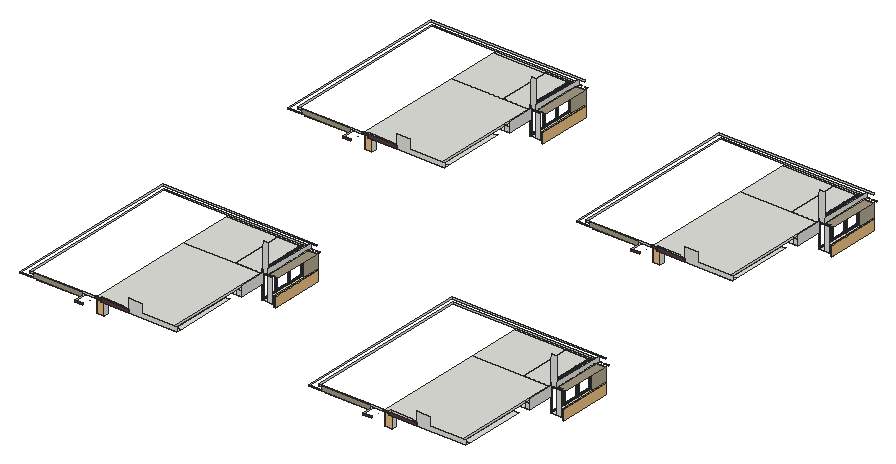
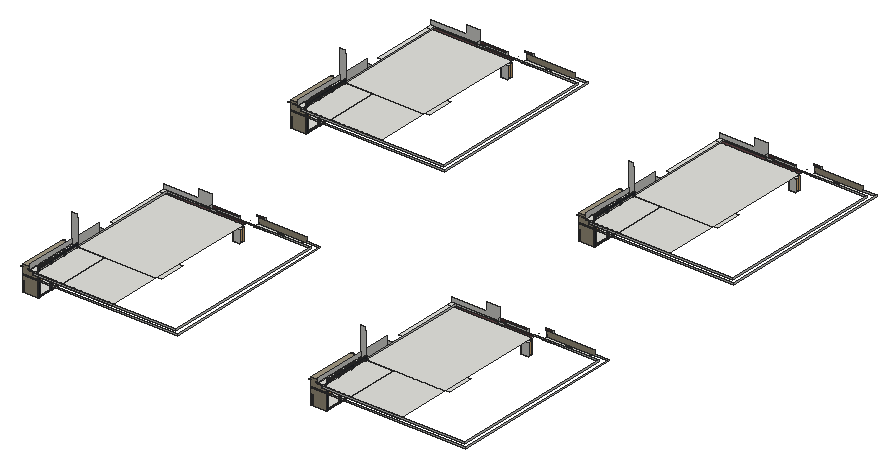
# SketchUp Ruby script. Lengths in inches.
U = 1.inch
M = Sketchup.active_model
def pt(a) = Geom::Point3d.new(a.map { |v| v * U })
def face(e, loops, mat)
  f = e.add_face(loops[0].map { |a| pt(a) })
  loops[1..].each { |l| e.add_face(l.map { |a| pt(a) }).erase! }
  f.material = f.back_material = mat if mat
  f
end
# faces: each face lists its corners as indices into pts; further lists are holes
def faces(e, pts, list, mat = nil) = list.each { |f| face(e, (f[0].is_a?(Array) ? f : [f]).map { |l| l.map { |i| pts[i] } }, mat) }
# xy, xz, yz: faces in a plane at the given z, y or x. An outline is a flat list of corners, or four numbers for a rectangle; further outlines are holes
def ring(l) = l.size == 4 ? [[l[0], l[1]], [l[2], l[1]], [l[2], l[3]], [l[0], l[3]]] : l.each_slice(2).to_a
def flat(e, list, mat, &to3) = list.each { |f| face(e, (f[0].is_a?(Array) ? f : [f]).map { |l| ring(l).map { |u, v| to3.(u, v) } }, mat) }
def xy(e, z, list, mat = nil) = flat(e, list, mat) { |x, y| [x, y, z] }
def xz(e, y, list, mat = nil) = flat(e, list, mat) { |x, z| [x, y, z] }
def yz(e, x, list, mat = nil) = flat(e, list, mat) { |y, z| [x, y, z] }
def lines(e, pts, list) = list.each { |a, b| e.add_line(pt(pts[a]), pt(pts[b])) }
# prism: a flat outline (further loops are holes) pulled along v
def prism(e, loops, v, mat = nil)
  f = face(e, loops, mat); d = Geom::Vector3d.new(v.map { |x| x * U })
  f.pushpull(f.normal.samedirection?(d) ? d.length : -d.length)
end
def box(e, o, s, mat = nil) = prism(e, [[o, [o[0] + s[0], o[1], o[2]], [o[0] + s[0], o[1] + s[1], o[2]], [o[0], o[1] + s[1], o[2]]]], [0, 0, s[2]], mat)
def at(x, y, z, deg = 0) = Geom::Transformation.translation(pt([x, y, z])) * Geom::Transformation.rotation(ORIGIN, Z_AXIS, deg.degrees)
def axes(o, x, y, z) = Geom::Transformation.new([*x, 0, *y, 0, *z, 0, *pt(o).to_a, 1])
def part(name) = M.definitions.add(name)
# library, detail: a bought-in or finely detailed component or shape, given as its bounding box
def library(name, o, s) = part(name).tap { |d| box(d.entities, o, s) }
def detail(e, o, s) = box(e.add_group.entities, o, s)
def put(e, d, t, mat = nil) = e.add_instance(d, t).tap { |i| i.material = mat if mat }
def group(e, t, mat = nil) = e.add_group.tap { |g| g.transformation = t; g.material = mat if mat }.entities
root = M.entities
M.materials.add("Wine2").color = [0, 0, 0]
M.materials["Wine2"].alpha = 0
M.materials.add("[0130_Gainsboro]").color = [39, 45, 50]
M.materials.add("[Concrete Tile]").color = [165, 155, 133]
M.materials.add("[Granite Brown]").color = [89, 59, 61]
c1 = part("Framed glazing panel")
xy(c1.entities,0,[[0,-0.98,43.07,0],[0,0,43.07,1.4]],"[0130_Gainsboro]")
xy(c1.entities,0.3,[[0.3,-1.43,42.77,-0.98]],"[0130_Gainsboro]")
xy(c1.entities,2.95,[[2.95,-1.43,40.12,-0.63],[2.95,-0.63,40.12,0],[2.95,0,40.12,0.64],[2.95,0.64,40.12,1.4]],"[0130_Gainsboro]")
xy(c1.entities,3.54,[[3.54,-0.63,39.53,0],[3.54,0,39.53,0.64]],"[0130_Gainsboro]")
xy(c1.entities,111.8125,[[3.54,-0.63,39.53,0],[3.54,0,39.53,0.64]],"[0130_Gainsboro]")
xy(c1.entities,112.4,[[2.95,-1.43,40.12,-0.63],[2.95,-0.63,40.12,0],[2.95,0,40.12,0.64],[2.95,0.64,40.12,1.4]],"[0130_Gainsboro]")
xy(c1.entities,115.05,[[0.3,-1.43,42.77,-0.98]],"[0130_Gainsboro]")
xy(c1.entities,115.35,[[0,-0.98,43.07,0],[0,0,43.07,1.4]],"[0130_Gainsboro]")
xz(c1.entities,-1.43,[[[0.3,0.3,42.77,115.05],[2.95,2.95,40.12,112.4]]],"[0130_Gainsboro]")
xz(c1.entities,-0.98,[[[0,0,43.07,115.35],[0.3,0.3,42.77,115.05]]],"[0130_Gainsboro]")
xz(c1.entities,-0.63,[[[2.95,2.95,40.12,112.4],[3.54,3.54,39.53,111.8125]]],"[0130_Gainsboro]")
xz(c1.entities,0,[[3.54,3.54,39.53,111.8125]],"Wine2")
xz(c1.entities,0,[[[0,0,43.07,115.35],[2.95,2.95,40.12,112.4]],[[2.95,2.95,40.12,112.4],[3.54,3.54,39.53,111.8125]]],"[0130_Gainsboro]")
xz(c1.entities,0.64,[[[2.95,2.95,40.12,112.4],[3.54,3.54,39.53,111.8125]]],"[0130_Gainsboro]")
xz(c1.entities,1.4,[[[0,0,43.07,115.35],[2.95,2.95,40.12,112.4]]],"[0130_Gainsboro]")
yz(c1.entities,0,[[-0.98,0,0,115.35],[0,0,1.4,115.35]],"[0130_Gainsboro]")
yz(c1.entities,0.3,[[-1.43,0.3,-0.98,115.05]],"[0130_Gainsboro]")
yz(c1.entities,2.95,[[-1.43,2.95,-0.63,112.4],[-0.63,2.95,0,112.4],[0,2.95,0.64,112.4],[0.64,2.95,1.4,112.4]],"[0130_Gainsboro]")
yz(c1.entities,3.54,[[-0.63,3.54,0,111.8125],[0,3.54,0.64,111.8125]],"[0130_Gainsboro]")
yz(c1.entities,39.53,[[-0.63,3.54,0,111.8125],[0,3.54,0.64,111.8125]],"[0130_Gainsboro]")
yz(c1.entities,40.12,[[-1.43,2.95,-0.63,112.4],[-0.63,2.95,0,112.4],[0,2.95,0.64,112.4],[0.64,2.95,1.4,112.4]],"[0130_Gainsboro]")
yz(c1.entities,42.77,[[-1.43,0.3,-0.98,115.05]],"[0130_Gainsboro]")
yz(c1.entities,43.07,[[-0.98,0,0,115.35],[0,0,1.4,115.35]],"[0130_Gainsboro]")
c2 = part("Glazed panel assembly")
put(c2.entities,c1,axes([90.57,1.43,0],[1.05148,0,0],[0,1,0],[0,0,1]))
put(c2.entities,c1,axes([0,1.43,0],[1.05148,0,0],[0,1,0],[0,0,1]))
put(c2.entities,c1,axes([45.29,1.43,0],[1.05148,0,0],[0,1,0],[0,0,1]))
c3 = library("Glass Railing",[0,0,0],[139.5,4.76,42])
c4 = library("Klein+raam",[128.36,12.7,0],[19.68,5.51,55.12])
xy(root,1538.8125,[[890.875,2295.875,954.6875,2505.21],[2109.0625,2295.875,2172.875,2505.21],[890.875,3710.5625,954.6875,3919.9],[2109.0625,3710.5625,2172.875,3919.9]])
xy(root,1575.17,[[557.88,1835.1875,588.66,1854.3125],[1776.07,1835.1875,1806.84,1854.3125],[557.88,3249.875,588.66,3269],[1776.07,3249.875,1806.84,3269]])
xy(root,1621.04,[[558.625,2156.01,913.875,2266.33],[1776.8125,2156.01,2132.0625,2266.33],[558.625,3570.7,913.875,3681.01],[1776.8125,3570.7,2132.0625,3681.01]])
xy(root,1627.45,[[557.88,1835.1875,588.66,1854.3125],[1776.07,1835.1875,1806.84,1854.3125],[557.88,3249.875,588.66,3269],[1776.07,3249.875,1806.84,3269]])
xy(root,1629.51,[[631.46,1835.1875,721.4,1873.375],[1849.65,1835.1875,1939.59,1873.375],[631.46,3249.875,721.4,3288.0625],[1849.65,3249.875,1939.59,3288.0625]])
xy(root,1638,[[333.68,1799.9375,333.68,1822.9375,406.8125,1822.9375,406.8125,1806.5625,442.15,1806.5625,442.15,1822.9375,523.04,1822.9375,523.04,1799.9375],[1551.87,1799.9375,1551.87,1822.9375,1625,1822.9375,1625,1806.5625,1660.33,1806.5625,1660.33,1822.9375,1741.23,1822.9375,1741.23,1799.9375],[431.33,1806.5625,442.15,1822.9375],[1649.52,1806.5625,1660.33,1822.9375],[709.36,1814.25,709.36,1822.9375,890.875,1822.9375,890.875,1835.1875,913.875,1835.1875,913.875,1814.25],
  [1927.54,1814.25,1927.54,1822.9375,2109.0625,1822.9375,2109.0625,1835.1875,2132.0625,1835.1875,2132.0625,1814.25],[557.88,1822.9375,558.625,1824.0625],[679.51,1822.9375,709.36,1827.125],[1776.07,1822.9375,1776.8125,1824.0625],[1897.7,1822.9375,1927.54,1827.125],
  [557.88,1824.0625,558.625,1835.1875],[1776.07,1824.0625,1776.8125,1835.1875],[558.625,1835.1875,890.875,2295.875],[894.3125,1835.1875,913.875,2094.15],[1776.8125,1835.1875,2109.0625,2295.875],
  [2112.5,1835.1875,2132.0625,2094.15],[558.625,2295.875,774.6875,2518.89],[774.6875,2295.875,890.875,2518.89],[890.875,2295.875,913.875,2505.21],[1776.8125,2295.875,1992.875,2518.89],
  [1992.875,2295.875,2109.0625,2518.89],[2109.0625,2295.875,2132.0625,2505.21],[890.875,2505.21,913.875,2518.89],[2109.0625,2505.21,2132.0625,2518.89],[558.625,2518.89,890.875,2531.375],
  [1776.8125,2518.89,2109.0625,2531.375],[333.68,3214.625,333.68,3237.625,406.8125,3237.625,406.8125,3221.25,442.15,3221.25,442.15,3237.625,523.04,3237.625,523.04,3214.625],[1551.87,3214.625,1551.87,3237.625,1625,3237.625,1625,3221.25,1660.33,3221.25,1660.33,3237.625,1741.23,3237.625,1741.23,3214.625],[431.33,3221.25,442.15,3237.625],[1649.52,3221.25,1660.33,3237.625],
  [709.36,3228.9375,709.36,3237.625,890.875,3237.625,890.875,3249.875,913.875,3249.875,913.875,3228.9375],[1927.54,3228.9375,1927.54,3237.625,2109.0625,3237.625,2109.0625,3249.875,2132.0625,3249.875,2132.0625,3228.9375],[557.88,3237.625,558.625,3238.75],[679.51,3237.625,709.36,3241.8125],[1776.07,3237.625,1776.8125,3238.75],
  [1897.7,3237.625,1927.54,3241.8125],[557.88,3238.75,558.625,3249.875],[1776.07,3238.75,1776.8125,3249.875],[558.625,3249.875,890.875,3710.5625],[894.3125,3249.875,913.875,3508.84],
  [1776.8125,3249.875,2109.0625,3710.5625],[2112.5,3249.875,2132.0625,3508.84],[558.625,3710.5625,774.6875,3933.57],[774.6875,3710.5625,890.875,3933.57],[890.875,3710.5625,913.875,3919.9],
  [1776.8125,3710.5625,1992.875,3933.57],[1992.875,3710.5625,2109.0625,3933.57],[2109.0625,3710.5625,2132.0625,3919.9],[890.875,3919.9,913.875,3933.57],[2109.0625,3919.9,2132.0625,3933.57],
  [558.625,3933.57,890.875,3946.0625],[1776.8125,3933.57,2109.0625,3946.0625]])
xy(root,1638,[[589.79,1814.25,709.36,1822.9375],[1807.98,1814.25,1927.54,1822.9375],[557.4,1822.9375,557.88,1824.0625],[709.36,1822.9375,890.875,1822.9375,890.875,1835.1875,558.625,1835.1875,558.625,1824.0625,679.51,1824.0625,679.51,1827.125,709.36,1827.125],[1775.59,1822.9375,1776.07,1824.0625],
  [1927.54,1822.9375,2109.0625,1822.9375,2109.0625,1835.1875,1776.8125,1835.1875,1776.8125,1824.0625,1897.7,1824.0625,1897.7,1827.125,1927.54,1827.125],[589.79,3228.9375,709.36,3237.625],[1807.98,3228.9375,1927.54,3237.625],[557.4,3237.625,557.88,3238.75],[709.36,3237.625,890.875,3237.625,890.875,3249.875,558.625,3249.875,558.625,3238.75,679.51,3238.75,679.51,3241.8125,709.36,3241.8125],
  [1775.59,3237.625,1776.07,3238.75],[1927.54,3237.625,2109.0625,3237.625,2109.0625,3249.875,1776.8125,3249.875,1776.8125,3238.75,1897.7,3238.75,1897.7,3241.8125,1927.54,3241.8125]],"[Granite Brown]")
xy(root,1639.25,[[774.6875,2295.875,890.875,2518.89],[1992.875,2295.875,2109.0625,2518.89],[774.6875,3710.5625,890.875,3933.57],[1992.875,3710.5625,2109.0625,3933.57]])
xy(root,1643.375,[[890.875,2295.875,913.875,2518.89],[2109.0625,2295.875,2132.0625,2518.89],[890.875,3710.5625,913.875,3933.57],[2109.0625,3710.5625,2132.0625,3933.57]])
xy(root,1643.375,[[913.875,2295.875,954.6875,2505.21],[2132.0625,2295.875,2172.875,2505.21],[913.875,3710.5625,954.6875,3919.9],[2132.0625,3710.5625,2172.875,3919.9]],"[Concrete Tile]")
xz(root,1763.25,[[523.04,1638,557.88,1644],[1741.23,1638,1776.07,1644]],"[Granite Brown]")
xz(root,1799.9375,[[262.875,1638,319.53,1644],[1481.0625,1638,1537.72,1644]])
xz(root,1799.9375,[[319.53,1638,523.04,1659.3125],[1537.72,1638,1741.23,1659.3125]],"[Concrete Tile]")
xz(root,1814.25,[[709.36,1638,913.875,1638,913.875,1656.6875,764.59,1656.6875,764.59,1693.1875,709.36,1693.1875],[1927.54,1638,2132.0625,1638,2132.0625,1656.6875,1982.78,1656.6875,1982.78,1693.1875,1927.54,1693.1875]])
xz(root,1814.25,[[589.79,1638,709.36,1650.875],[1807.98,1638,1927.54,1650.875]],"[Granite Brown]")
xz(root,1822.9375,[[285.875,1638,557.4,1644],[589.79,1638,679.51,1650.875],[679.51,1638,709.36,1644],[709.36,1638,890.875,1644],[1504.0625,1638,1775.59,1644],
  [1807.98,1638,1897.7,1650.875],[1897.7,1638,1927.54,1644],[1927.54,1638,2109.0625,1644]])
xz(root,1822.9375,[[557.4,1638,557.88,1644],[1775.59,1638,1776.07,1644]],"[Granite Brown]")
xz(root,1824.0625,[[557.4,1638,679.51,1644],[1775.59,1638,1897.7,1644]],"[Granite Brown]")
xz(root,1827.125,[[679.51,1638,709.36,1644],[1897.7,1638,1927.54,1644]])
xz(root,1854.3125,[[557.88,1575.17,588.66,1627.45],[1776.07,1575.17,1806.84,1627.45]])
xz(root,2156.01,[[894.3125,1621.04,913.875,1644],[2112.5,1621.04,2132.0625,1644]])
xz(root,2295.875,[[913.875,1538.8125,930.75,1638],[2132.0625,1538.8125,2148.9375,1638],[774.6875,1638,890.875,1639.25],[913.875,1638,930.75,1643.375],[1992.875,1638,2109.0625,1639.25],
  [2132.0625,1638,2148.9375,1643.375],[890.875,1643.375,913.875,1643.375,913.875,1764,894.3125,1764,894.3125,1749.375,890.875,1749.375],[913.875,1643.375,930.75,1644],[930.75,1643.375,954.6875,1644],[2109.0625,1643.375,2132.0625,1643.375,2132.0625,1764,2112.5,1764,2112.5,1749.375,2109.0625,1749.375],
  [2132.0625,1643.375,2148.9375,1644],[2148.9375,1643.375,2172.875,1644]])
xz(root,2505.21,[[890.875,1538.8125,954.6875,1538.8125,954.6875,1643.375,913.875,1643.375,913.875,1638,890.875,1638],[2109.0625,1538.8125,2172.875,1538.8125,2172.875,1643.375,2132.0625,1643.375,2132.0625,1638,2109.0625,1638]],"[Concrete Tile]")
xz(root,2518.89,[[774.6875,1638,890.875,1639.25],[1992.875,1638,2109.0625,1639.25],[913.875,1643.375,954.6875,1644],[2132.0625,1643.375,2172.875,1644]])
xz(root,2531.375,[[285.875,1638,890.875,1644],[1504.0625,1638,2109.0625,1644]])
xz(root,2554.375,[[262.875,1638,913.875,1644],[1481.0625,1638,2132.0625,1644]])
xz(root,3177.9375,[[523.04,1638,557.88,1644],[1741.23,1638,1776.07,1644]],"[Granite Brown]")
xz(root,3214.625,[[262.875,1638,319.53,1644],[1481.0625,1638,1537.72,1644]])
xz(root,3214.625,[[319.53,1638,523.04,1659.3125],[1537.72,1638,1741.23,1659.3125]],"[Concrete Tile]")
xz(root,3228.9375,[[709.36,1638,913.875,1638,913.875,1656.6875,764.59,1656.6875,764.59,1693.1875,709.36,1693.1875],[1927.54,1638,2132.0625,1638,2132.0625,1656.6875,1982.78,1656.6875,1982.78,1693.1875,1927.54,1693.1875]])
xz(root,3228.9375,[[589.79,1638,709.36,1650.875],[1807.98,1638,1927.54,1650.875]],"[Granite Brown]")
xz(root,3237.625,[[285.875,1638,557.4,1644],[589.79,1638,679.51,1650.875],[679.51,1638,709.36,1644],[709.36,1638,890.875,1644],[1504.0625,1638,1775.59,1644],
  [1807.98,1638,1897.7,1650.875],[1897.7,1638,1927.54,1644],[1927.54,1638,2109.0625,1644]])
xz(root,3237.625,[[557.4,1638,557.88,1644],[1775.59,1638,1776.07,1644]],"[Granite Brown]")
xz(root,3238.75,[[557.4,1638,679.51,1644],[1775.59,1638,1897.7,1644]],"[Granite Brown]")
xz(root,3241.8125,[[679.51,1638,709.36,1644],[1897.7,1638,1927.54,1644]])
xz(root,3269,[[557.88,1575.17,588.66,1627.45],[1776.07,1575.17,1806.84,1627.45]])
xz(root,3570.7,[[894.3125,1621.04,913.875,1644],[2112.5,1621.04,2132.0625,1644]])
xz(root,3710.5625,[[913.875,1538.8125,930.75,1638],[2132.0625,1538.8125,2148.9375,1638],[774.6875,1638,890.875,1639.25],[913.875,1638,930.75,1643.375],[1992.875,1638,2109.0625,1639.25],
  [2132.0625,1638,2148.9375,1643.375],[890.875,1643.375,913.875,1643.375,913.875,1764,894.3125,1764,894.3125,1749.375,890.875,1749.375],[913.875,1643.375,930.75,1644],[930.75,1643.375,954.6875,1644],[2109.0625,1643.375,2132.0625,1643.375,2132.0625,1764,2112.5,1764,2112.5,1749.375,2109.0625,1749.375],
  [2132.0625,1643.375,2148.9375,1644],[2148.9375,1643.375,2172.875,1644]])
xz(root,3919.9,[[890.875,1538.8125,954.6875,1538.8125,954.6875,1643.375,913.875,1643.375,913.875,1638,890.875,1638],[2109.0625,1538.8125,2172.875,1538.8125,2172.875,1643.375,2132.0625,1643.375,2132.0625,1638,2109.0625,1638]],"[Concrete Tile]")
xz(root,3933.57,[[774.6875,1638,890.875,1639.25],[1992.875,1638,2109.0625,1639.25],[913.875,1643.375,954.6875,1644],[2132.0625,1643.375,2172.875,1644]])
xz(root,3946.0625,[[285.875,1638,890.875,1644],[1504.0625,1638,2109.0625,1644]])
xz(root,3969.0625,[[262.875,1638,913.875,1644],[1481.0625,1638,2132.0625,1644]])
yz(root,262.875,[[1799.9375,1638,2554.375,1644],[3214.625,1638,3969.0625,1644]])
yz(root,285.875,[[1822.9375,1638,2531.375,1644],[3237.625,1638,3946.0625,1644]])
yz(root,523.04,[[1763.25,1638,1799.9375,1644],[3177.9375,1638,3214.625,1644]])
yz(root,557.4,[[1822.9375,1638,1824.0625,1644],[3237.625,1638,3238.75,1644]])
yz(root,588.66,[[1835.1875,1575.17,1854.3125,1627.45],[3249.875,1575.17,3269,1627.45]])
yz(root,589.79,[[1814.25,1638,1822.9375,1650.875],[3228.9375,1638,3237.625,1650.875]])
yz(root,679.51,[[1822.9375,1638,1824.0625,1644],[1824.0625,1638,1827.125,1644],[3237.625,1638,3238.75,1644],[3238.75,1638,3241.8125,1644]])
yz(root,709.36,[[1814.25,1638,1822.9375,1650.875],[1822.9375,1638,1827.125,1644],[3228.9375,1638,3237.625,1650.875],[3237.625,1638,3241.8125,1644]])
yz(root,774.6875,[[2295.875,1638,2518.89,1639.25],[3710.5625,1638,3933.57,1639.25]])
yz(root,890.875,[[1822.9375,1638,1822.9375,1644,2295.875,1644,2295.875,1643.375,2518.89,1643.375,2518.89,1644,2531.375,1644,2531.375,1638,2518.89,1638,2518.89,1639.25,2295.875,1639.25,2295.875,1638],[2295.875,1638,2505.21,1639.25],[2505.21,1638,2518.89,1639.25],[3237.625,1638,3237.625,1644,3710.5625,1644,3710.5625,1643.375,3933.57,1643.375,3933.57,1644,3946.0625,1644,3946.0625,1638,3933.57,1638,3933.57,1639.25,3710.5625,1639.25,3710.5625,1638],[3710.5625,1638,3919.9,1639.25],
  [3919.9,1638,3933.57,1639.25],[2295.875,1643.375,2518.89,1644],[3710.5625,1643.375,3933.57,1644]])
yz(root,913.875,[[2156.01,1621.04,2266.33,1661.36],[3570.7,1621.04,3681.01,1661.36],[2295.875,1638,2505.21,1643.375],[2505.21,1638,2518.89,1643.375],[3710.5625,1638,3919.9,1643.375],
  [3919.9,1638,3933.57,1643.375],[2295.875,1643.375,2518.89,1663.0625],[3710.5625,1643.375,3933.57,1663.0625]])
yz(root,1481.0625,[[1799.9375,1638,2554.375,1644],[3214.625,1638,3969.0625,1644]])
yz(root,1504.0625,[[1822.9375,1638,2531.375,1644],[3237.625,1638,3946.0625,1644]])
yz(root,1741.23,[[1763.25,1638,1799.9375,1644],[3177.9375,1638,3214.625,1644]])
yz(root,1775.59,[[1822.9375,1638,1824.0625,1644],[3237.625,1638,3238.75,1644]])
yz(root,1806.84,[[1835.1875,1575.17,1854.3125,1627.45],[3249.875,1575.17,3269,1627.45]])
yz(root,1807.98,[[1814.25,1638,1822.9375,1650.875],[3228.9375,1638,3237.625,1650.875]])
yz(root,1897.7,[[1822.9375,1638,1824.0625,1644],[1824.0625,1638,1827.125,1644],[3237.625,1638,3238.75,1644],[3238.75,1638,3241.8125,1644]])
yz(root,1927.54,[[1814.25,1638,1822.9375,1650.875],[1822.9375,1638,1827.125,1644],[3228.9375,1638,3237.625,1650.875],[3237.625,1638,3241.8125,1644]])
yz(root,1992.875,[[2295.875,1638,2518.89,1639.25],[3710.5625,1638,3933.57,1639.25]])
yz(root,2109.0625,[[1822.9375,1638,1822.9375,1644,2295.875,1644,2295.875,1643.375,2518.89,1643.375,2518.89,1644,2531.375,1644,2531.375,1638,2518.89,1638,2518.89,1639.25,2295.875,1639.25,2295.875,1638],[2295.875,1638,2505.21,1639.25],[2505.21,1638,2518.89,1639.25],[3237.625,1638,3237.625,1644,3710.5625,1644,3710.5625,1643.375,3933.57,1643.375,3933.57,1644,3946.0625,1644,3946.0625,1638,3933.57,1638,3933.57,1639.25,3710.5625,1639.25,3710.5625,1638],[3710.5625,1638,3919.9,1639.25],
  [3919.9,1638,3933.57,1639.25],[2295.875,1643.375,2518.89,1644],[3710.5625,1643.375,3933.57,1644]])
yz(root,2132.0625,[[2156.01,1621.04,2266.33,1661.36],[3570.7,1621.04,3681.01,1661.36],[2295.875,1638,2505.21,1643.375],[2505.21,1638,2518.89,1643.375],[3710.5625,1638,3919.9,1643.375],
  [3919.9,1638,3933.57,1643.375],[2295.875,1643.375,2518.89,1663.0625],[3710.5625,1643.375,3933.57,1663.0625]])
p = [[1774.53,1835.1875,1575.17],[1775.59,1835.1875,1575.17],[1775.59,1835.1875,1627.45],[1774.53,1835.1875,1627.45],[1775.59,1798.5625,1638],[1776.8125,1798.5625,1638],
  [556.34,1835.1875,1575.17],[557.4,1835.1875,1575.17],[557.4,1835.1875,1627.45],[556.34,1835.1875,1627.45],[557.4,1798.5625,1638],[558.625,1798.5625,1638],
  [1775.59,3249.875,1627.45],[1774.53,3249.875,1627.45],[1774.53,3249.875,1575.17],[1775.59,3249.875,1575.17],[1775.59,3213.25,1638],[1776.8125,3213.25,1638],
  [556.34,3249.875,1575.17],[557.4,3249.875,1575.17],[557.4,3249.875,1627.45],[556.34,3249.875,1627.45],[557.4,3213.25,1638],[558.625,3213.25,1638]]
lines(root,p,[[0,1],[2,3],[0,3],[4,5],[6,7],[8,9],[6,9],[10,11],[12,13],[14,15],[14,13],[16,17],
  [18,19],[20,21],[18,21],[22,23]])
put(root,c2,axes([2109.0625,2295.875,1538.8125],[0,1.54079,0],[-1,0,0],[0,0,1]))
put(root,c2,axes([890.875,2295.875,1538.8125],[0,1.54079,0],[-1,0,0],[0,0,1]))
put(root,c2,axes([2109.0625,3710.5625,1538.8125],[0,1.54079,0],[-1,0,0],[0,0,1]))
put(root,c2,axes([890.875,3710.5625,1538.8125],[0,1.54079,0],[-1,0,0],[0,0,1]))
put(root,c3,axes([2172.875,2282.01,1538.8125],[0,1.6,0],[-1,0,0],[0,0,1]))
put(root,c3,axes([954.6875,2282.01,1538.8125],[0,1.6,0],[-1,0,0],[0,0,1]))
put(root,c3,axes([2172.875,3696.7,1538.8125],[0,1.6,0],[-1,0,0],[0,0,1]))
put(root,c3,axes([954.6875,3696.7,1538.8125],[0,1.6,0],[-1,0,0],[0,0,1]))
put(root,c4,axes([1571.78,1826.29,1575.17],[1.58777,0,0],[0,0.68,0],[0,0,0.99202]))
put(root,c4,axes([353.6,1826.29,1575.17],[1.58777,0,0],[0,0.68,0],[0,0,0.99202]))
put(root,c4,axes([1571.78,3240.97,1575.17],[1.58777,0,0],[0,0.68,0],[0,0,0.99202]))
put(root,c4,axes([353.6,3240.97,1575.17],[1.58777,0,0],[0,0.68,0],[0,0,0.99202]))
